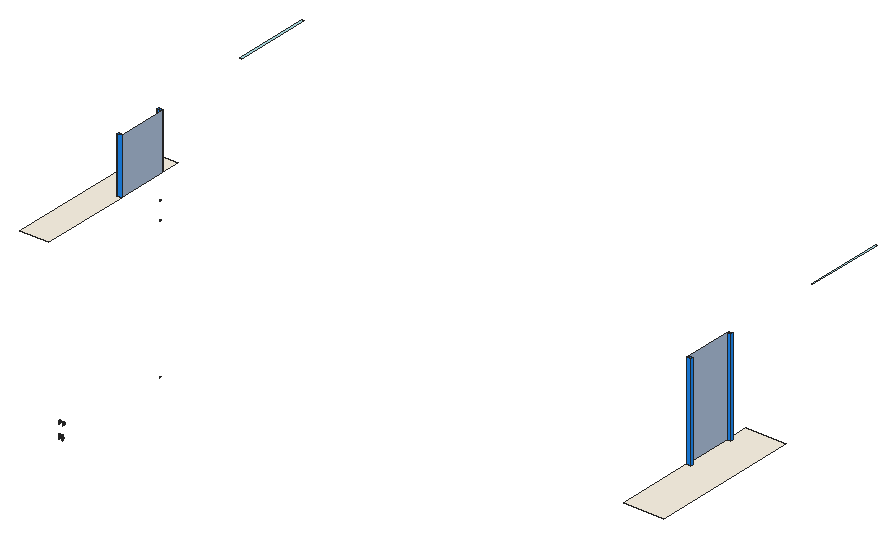
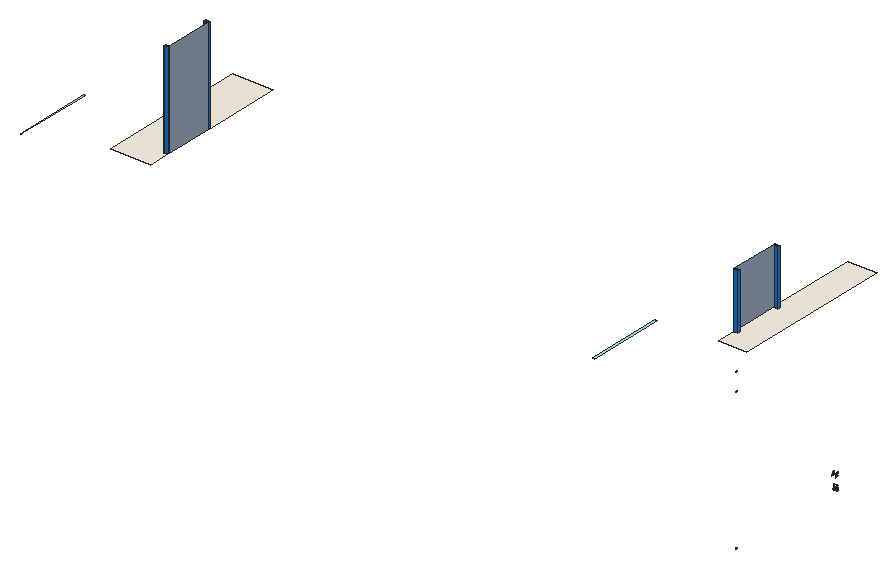
# SketchUp Ruby script. Lengths in inches.
U = 1.inch
M = Sketchup.active_model
def pt(a) = Geom::Point3d.new(a.map { |v| v * U })
def face(e, loops, mat)
  f = e.add_face(loops[0].map { |a| pt(a) })
  loops[1..].each { |l| e.add_face(l.map { |a| pt(a) }).erase! }
  f.material = f.back_material = mat if mat
  f
end
# faces: each face lists its corners as indices into pts; further lists are holes
def faces(e, pts, list, mat = nil) = list.each { |f| face(e, (f[0].is_a?(Array) ? f : [f]).map { |l| l.map { |i| pts[i] } }, mat) }
# xy, xz, yz: faces in a plane at the given z, y or x. An outline is a flat list of corners, or four numbers for a rectangle; further outlines are holes
def ring(l) = l.size == 4 ? [[l[0], l[1]], [l[2], l[1]], [l[2], l[3]], [l[0], l[3]]] : l.each_slice(2).to_a
def flat(e, list, mat, &to3) = list.each { |f| face(e, (f[0].is_a?(Array) ? f : [f]).map { |l| ring(l).map { |u, v| to3.(u, v) } }, mat) }
def xy(e, z, list, mat = nil) = flat(e, list, mat) { |x, y| [x, y, z] }
def xz(e, y, list, mat = nil) = flat(e, list, mat) { |x, z| [x, y, z] }
def yz(e, x, list, mat = nil) = flat(e, list, mat) { |y, z| [x, y, z] }
def lines(e, pts, list) = list.each { |a, b| e.add_line(pt(pts[a]), pt(pts[b])) }
# prism: a flat outline (further loops are holes) pulled along v
def prism(e, loops, v, mat = nil)
  f = face(e, loops, mat); d = Geom::Vector3d.new(v.map { |x| x * U })
  f.pushpull(f.normal.samedirection?(d) ? d.length : -d.length)
end
def box(e, o, s, mat = nil) = prism(e, [[o, [o[0] + s[0], o[1], o[2]], [o[0] + s[0], o[1] + s[1], o[2]], [o[0], o[1] + s[1], o[2]]]], [0, 0, s[2]], mat)
def at(x, y, z, deg = 0) = Geom::Transformation.translation(pt([x, y, z])) * Geom::Transformation.rotation(ORIGIN, Z_AXIS, deg.degrees)
def axes(o, x, y, z) = Geom::Transformation.new([*x, 0, *y, 0, *z, 0, *pt(o).to_a, 1])
def part(name) = M.definitions.add(name)
# library, detail: a bought-in or finely detailed component or shape, given as its bounding box
def library(name, o, s) = part(name).tap { |d| box(d.entities, o, s) }
def detail(e, o, s) = box(e.add_group.entities, o, s)
def put(e, d, t, mat = nil) = e.add_instance(d, t).tap { |i| i.material = mat if mat }
def group(e, t, mat = nil) = e.add_group.tap { |g| g.transformation = t; g.material = mat if mat }.entities
root = M.entities
M.materials.add("Material \#1").color = [140, 140, 140]
M.materials.add("[0030_OldLace]").color = [253, 245, 230]
M.materials.add("[0094_PowderBlue]").color = [176, 224, 230]
M.materials.add("[0098_DodgerBlue]").color = [30, 144, 255]
M.materials.add("[0099_LightSteelBlue]").color = [176, 196, 222]
xy(root,58.6641,[[266.1811,291.2578,266.1811,291.2765,266.1568,291.2691],[266.1811,291.2578,266.203,291.2867,266.1811,291.2765],[266.1811,291.2578,266.2055,291.2691,266.203,291.2867],[266.1568,291.2691,266.1593,291.2867,266.1355,291.3016],[266.1568,291.2691,266.1811,291.2765,266.1593,291.2867],
  [266.2055,291.2691,266.2223,291.316,266.203,291.2867],[266.2055,291.2691,266.2268,291.3016,266.2223,291.316],[266.1593,291.2867,266.14,291.316,266.1355,291.3016],[266.1355,291.3016,266.14,291.316,266.1196,291.3515],[266.2268,291.3016,266.2366,291.3609,266.2223,291.316],
  [266.2268,291.3016,266.2427,291.3515,266.2366,291.3609],[266.14,291.316,266.1257,291.3609,266.1196,291.3515],[266.1196,291.3515,266.1257,291.3609,266.1111,291.4127],[266.2427,291.3515,266.2441,291.4159,266.2366,291.3609],[266.2427,291.3515,266.2512,291.4127,266.2441,291.4159],
  [266.1257,291.3609,266.1181,291.4159,266.1111,291.4127],[266.1111,291.4127,266.1181,291.4159,266.1111,291.4778],[266.2512,291.4127,266.2442,291.4745,266.2441,291.4159],[266.2512,291.4127,266.2512,291.4778,266.2442,291.4745],[266.1181,291.4159,266.1181,291.4745,266.1111,291.4778],
  [266.1181,291.4745,266.1196,291.539,266.1111,291.4778],[266.1181,291.4745,266.1257,291.5296,266.1196,291.539],[266.2442,291.4745,266.2512,291.4778,266.2366,291.5296],[266.2512,291.4778,266.2427,291.539,266.2366,291.5296],[266.1257,291.5296,266.1355,291.5888,266.1196,291.539],
  [266.1257,291.5296,266.14,291.5745,266.1355,291.5888],[266.2366,291.5296,266.2427,291.539,266.2223,291.5745],[266.2427,291.539,266.2268,291.5888,266.2223,291.5745],[266.14,291.5745,266.1568,291.6214,266.1355,291.5888],[266.14,291.5745,266.1593,291.6038,266.1568,291.6214],
  [266.2223,291.5745,266.2268,291.5888,266.203,291.6038],[266.2268,291.5888,266.2055,291.6214,266.203,291.6038],[266.1593,291.6038,266.1811,291.6327,266.1568,291.6214],[266.1593,291.6038,266.1811,291.6139,266.1811,291.6327],[266.203,291.6038,266.2055,291.6214,266.1811,291.6139],
  [266.1811,291.6139,266.2055,291.6214,266.1811,291.6327]],"Material \#1")
xy(root,58.6839,[[266.1811,291.2578,266.1568,291.2691,266.1593,291.2867],[266.1811,291.2578,266.1593,291.2867,266.1811,291.2765],[266.1811,291.2578,266.1811,291.2765,266.2055,291.2691],[266.1568,291.2691,266.1355,291.3016,266.14,291.316],[266.1568,291.2691,266.14,291.316,266.1593,291.2867],
  [266.2055,291.2691,266.1811,291.2765,266.203,291.2867],[266.2055,291.2691,266.203,291.2867,266.2268,291.3016],[266.203,291.2867,266.2223,291.316,266.2268,291.3016],[266.1355,291.3016,266.1196,291.3515,266.1257,291.3609],[266.1355,291.3016,266.1257,291.3609,266.14,291.316],
  [266.2268,291.3016,266.2223,291.316,266.2427,291.3515],[266.2223,291.316,266.2366,291.3609,266.2427,291.3515],[266.1196,291.3515,266.1111,291.4127,266.1181,291.4159],[266.1196,291.3515,266.1181,291.4159,266.1257,291.3609],[266.2427,291.3515,266.2366,291.3609,266.2512,291.4127],
  [266.2366,291.3609,266.2441,291.4159,266.2512,291.4127],[266.1111,291.4127,266.1111,291.4778,266.1181,291.4745],[266.1111,291.4127,266.1181,291.4745,266.1181,291.4159],[266.2512,291.4127,266.2441,291.4159,266.2512,291.4778],[266.2441,291.4159,266.2442,291.4745,266.2512,291.4778],
  [266.1181,291.4745,266.1111,291.4778,266.1257,291.5296],[266.2442,291.4745,266.2366,291.5296,266.2427,291.539],[266.2442,291.4745,266.2427,291.539,266.2512,291.4778],[266.1111,291.4778,266.1196,291.539,266.1257,291.5296],[266.1257,291.5296,266.1196,291.539,266.14,291.5745],
  [266.2366,291.5296,266.2223,291.5745,266.2268,291.5888],[266.2366,291.5296,266.2268,291.5888,266.2427,291.539],[266.1196,291.539,266.1355,291.5888,266.14,291.5745],[266.14,291.5745,266.1355,291.5888,266.1593,291.6038],[266.2223,291.5745,266.203,291.6038,266.2055,291.6214],
  [266.2223,291.5745,266.2055,291.6214,266.2268,291.5888],[266.1355,291.5888,266.1568,291.6214,266.1593,291.6038],[266.1593,291.6038,266.1568,291.6214,266.1811,291.6139],[266.203,291.6038,266.1811,291.6139,266.1811,291.6327],[266.203,291.6038,266.1811,291.6327,266.2055,291.6214],
  [266.1811,291.6139,266.1568,291.6214,266.1811,291.6327]],"Material \#1")
xy(root,93.8273,[[266.1811,291.2578,266.1593,291.2867,266.1568,291.2691],[266.1811,291.2578,266.1811,291.2765,266.1593,291.2867],[266.1811,291.2578,266.2055,291.2691,266.1811,291.2765],[266.1568,291.2691,266.14,291.316,266.1355,291.3016],[266.1568,291.2691,266.1593,291.2867,266.14,291.316],
  [266.2055,291.2691,266.203,291.2867,266.1811,291.2765],[266.2055,291.2691,266.2268,291.3016,266.203,291.2867],[266.203,291.2867,266.2268,291.3016,266.2223,291.316],[266.1355,291.3016,266.1257,291.3609,266.1196,291.3515],[266.1355,291.3016,266.14,291.316,266.1257,291.3609],
  [266.2268,291.3016,266.2427,291.3515,266.2223,291.316],[266.2223,291.316,266.2427,291.3515,266.2365,291.3609],[266.1196,291.3515,266.1181,291.4159,266.1111,291.4127],[266.1196,291.3515,266.1257,291.3609,266.1181,291.4159],[266.2427,291.3515,266.2511,291.4127,266.2365,291.3609],
  [266.2365,291.3609,266.2511,291.4127,266.2441,291.4159],[266.1111,291.4127,266.1181,291.4159,266.1181,291.4745],[266.1111,291.4127,266.1181,291.4745,266.1111,291.4778],[266.2511,291.4127,266.2511,291.4778,266.2441,291.4159],[266.2441,291.4159,266.2511,291.4778,266.2441,291.4745],
  [266.1181,291.4745,266.1257,291.5296,266.1111,291.4778],[266.2441,291.4745,266.2427,291.539,266.2365,291.5296],[266.2441,291.4745,266.2511,291.4778,266.2427,291.539],[266.1111,291.4778,266.1257,291.5296,266.1196,291.539],[266.1257,291.5296,266.14,291.5745,266.1196,291.539],
  [266.2365,291.5296,266.2268,291.5888,266.2223,291.5745],[266.2365,291.5296,266.2427,291.539,266.2268,291.5888],[266.1196,291.539,266.14,291.5745,266.1355,291.5888],[266.14,291.5745,266.1593,291.6038,266.1355,291.5888],[266.2223,291.5745,266.2055,291.6214,266.203,291.6038],
  [266.2223,291.5745,266.2268,291.5888,266.2055,291.6214],[266.1355,291.5888,266.1593,291.6038,266.1568,291.6214],[266.1593,291.6038,266.1811,291.6139,266.1568,291.6214],[266.203,291.6038,266.1811,291.6327,266.1811,291.6139],[266.203,291.6038,266.2055,291.6214,266.1811,291.6327],
  [266.1811,291.6139,266.1811,291.6327,266.1568,291.6214]],"Material \#1")
xy(root,93.8471,[[266.1811,291.2578,266.1568,291.2691,266.1811,291.2765],[266.1811,291.2578,266.1811,291.2765,266.203,291.2867],[266.1811,291.2578,266.203,291.2867,266.2055,291.2691],[266.1568,291.2691,266.1355,291.3016,266.1593,291.2867],[266.1568,291.2691,266.1593,291.2867,266.1811,291.2765],
  [266.2055,291.2691,266.203,291.2867,266.2223,291.316],[266.2055,291.2691,266.2223,291.316,266.2268,291.3016],[266.1593,291.2867,266.1355,291.3016,266.14,291.316],[266.1355,291.3016,266.1196,291.3515,266.14,291.316],[266.2268,291.3016,266.2223,291.316,266.2365,291.3609],
  [266.2268,291.3016,266.2365,291.3609,266.2427,291.3515],[266.14,291.316,266.1196,291.3515,266.1257,291.3609],[266.1196,291.3515,266.1111,291.4127,266.1257,291.3609],[266.2427,291.3515,266.2365,291.3609,266.2441,291.4159],[266.2427,291.3515,266.2441,291.4159,266.2511,291.4127],
  [266.1257,291.3609,266.1111,291.4127,266.1181,291.4159],[266.1111,291.4127,266.1111,291.4778,266.1181,291.4159],[266.2511,291.4127,266.2441,291.4159,266.2441,291.4745],[266.2511,291.4127,266.2441,291.4745,266.2511,291.4778],[266.1181,291.4159,266.1111,291.4778,266.1181,291.4745],
  [266.1181,291.4745,266.1111,291.4778,266.1196,291.539],[266.1181,291.4745,266.1196,291.539,266.1257,291.5296],[266.2441,291.4745,266.2365,291.5296,266.2511,291.4778],[266.2511,291.4778,266.2365,291.5296,266.2427,291.539],[266.1257,291.5296,266.1196,291.539,266.1355,291.5888],
  [266.1257,291.5296,266.1355,291.5888,266.14,291.5745],[266.2365,291.5296,266.2223,291.5745,266.2427,291.539],[266.2427,291.539,266.2223,291.5745,266.2268,291.5888],[266.14,291.5745,266.1355,291.5888,266.1568,291.6214],[266.14,291.5745,266.1568,291.6214,266.1593,291.6038],
  [266.2223,291.5745,266.203,291.6038,266.2268,291.5888],[266.2268,291.5888,266.203,291.6038,266.2055,291.6214],[266.1593,291.6038,266.1568,291.6214,266.1811,291.6327],[266.1593,291.6038,266.1811,291.6327,266.1811,291.6139],[266.203,291.6038,266.1811,291.6139,266.2055,291.6214],
  [266.1811,291.6139,266.1811,291.6327,266.2055,291.6214]],"Material \#1")
xy(root,96,[[410,257.0899,410,276.9647,411,276.9647,411,277.4688,410,277.4688,410,289.4649,411,289.4649,411,289.9649,410,289.9649,410,295.4649,420,295.4649,420,257.0899]],"[0030_OldLace]")
xy(root,98.2902,[[266.1811,291.2578,266.1811,291.2765,266.1568,291.2691],[266.1811,291.2578,266.203,291.2867,266.1811,291.2765],[266.1811,291.2578,266.2055,291.2691,266.203,291.2867],[266.1568,291.2691,266.1593,291.2867,266.1355,291.3016],[266.1568,291.2691,266.1811,291.2765,266.1593,291.2867],
  [266.2055,291.2691,266.2223,291.316,266.203,291.2867],[266.2055,291.2691,266.2268,291.3016,266.2223,291.316],[266.1593,291.2867,266.14,291.316,266.1355,291.3016],[266.1355,291.3016,266.14,291.316,266.1196,291.3515],[266.2268,291.3016,266.2365,291.3609,266.2223,291.316],
  [266.2268,291.3016,266.2427,291.3515,266.2365,291.3609],[266.14,291.316,266.1257,291.3609,266.1196,291.3515],[266.1196,291.3515,266.1257,291.3609,266.1111,291.4127],[266.2427,291.3515,266.2441,291.4159,266.2365,291.3609],[266.2427,291.3515,266.2511,291.4127,266.2441,291.4159],
  [266.1257,291.3609,266.1181,291.4159,266.1111,291.4127],[266.1111,291.4127,266.1181,291.4159,266.1111,291.4778],[266.2511,291.4127,266.2441,291.4745,266.2441,291.4159],[266.2511,291.4127,266.2511,291.4778,266.2441,291.4745],[266.1181,291.4159,266.1181,291.4745,266.1111,291.4778],
  [266.1181,291.4745,266.1196,291.539,266.1111,291.4778],[266.1181,291.4745,266.1257,291.5296,266.1196,291.539],[266.2441,291.4745,266.2511,291.4778,266.2365,291.5296],[266.2511,291.4778,266.2427,291.539,266.2365,291.5296],[266.1257,291.5296,266.1355,291.5888,266.1196,291.539],
  [266.1257,291.5296,266.14,291.5745,266.1355,291.5888],[266.2365,291.5296,266.2427,291.539,266.2223,291.5745],[266.2427,291.539,266.2268,291.5888,266.2223,291.5745],[266.14,291.5745,266.1568,291.6214,266.1355,291.5888],[266.14,291.5745,266.1593,291.6038,266.1568,291.6214],
  [266.2223,291.5745,266.2268,291.5888,266.203,291.6038],[266.2268,291.5888,266.2055,291.6214,266.203,291.6038],[266.1593,291.6038,266.1811,291.6327,266.1568,291.6214],[266.1593,291.6038,266.1811,291.6139,266.1811,291.6327],[266.203,291.6038,266.2055,291.6214,266.1811,291.6139],
  [266.1811,291.6139,266.2055,291.6214,266.1811,291.6327]],"Material \#1")
xy(root,98.3101,[[266.1811,291.2578,266.1568,291.2691,266.1593,291.2867],[266.1811,291.2578,266.1593,291.2867,266.1811,291.2765],[266.1811,291.2578,266.1811,291.2765,266.2055,291.2691],[266.1568,291.2691,266.1355,291.3016,266.14,291.316],[266.1568,291.2691,266.14,291.316,266.1593,291.2867],
  [266.2055,291.2691,266.1811,291.2765,266.203,291.2867],[266.2055,291.2691,266.203,291.2867,266.2268,291.3016],[266.203,291.2867,266.2223,291.316,266.2268,291.3016],[266.1355,291.3016,266.1196,291.3515,266.1257,291.3609],[266.1355,291.3016,266.1257,291.3609,266.14,291.316],
  [266.2268,291.3016,266.2223,291.316,266.2427,291.3515],[266.2223,291.316,266.2365,291.3609,266.2427,291.3515],[266.1196,291.3515,266.1111,291.4127,266.1181,291.4159],[266.1196,291.3515,266.1181,291.4159,266.1257,291.3609],[266.2427,291.3515,266.2365,291.3609,266.2511,291.4127],
  [266.2365,291.3609,266.2441,291.4159,266.2511,291.4127],[266.1111,291.4127,266.1111,291.4778,266.1181,291.4745],[266.1111,291.4127,266.1181,291.4745,266.1181,291.4159],[266.2511,291.4127,266.2441,291.4159,266.2511,291.4778],[266.2441,291.4159,266.2441,291.4745,266.2511,291.4778],
  [266.1181,291.4745,266.1111,291.4778,266.1257,291.5296],[266.2441,291.4745,266.2365,291.5296,266.2427,291.539],[266.2441,291.4745,266.2427,291.539,266.2511,291.4778],[266.1111,291.4778,266.1196,291.539,266.1257,291.5296],[266.1257,291.5296,266.1196,291.539,266.14,291.5745],
  [266.2365,291.5296,266.2223,291.5745,266.2268,291.5888],[266.2365,291.5296,266.2268,291.5888,266.2427,291.539],[266.1196,291.539,266.1355,291.5888,266.14,291.5745],[266.14,291.5745,266.1355,291.5888,266.1593,291.6038],[266.2223,291.5745,266.203,291.6038,266.2055,291.6214],
  [266.2223,291.5745,266.2055,291.6214,266.2268,291.5888],[266.1355,291.5888,266.1568,291.6214,266.1593,291.6038],[266.1593,291.6038,266.1568,291.6214,266.1811,291.6139],[266.203,291.6038,266.1811,291.6139,266.1811,291.6327],[266.203,291.6038,266.1811,291.6327,266.2055,291.6214],
  [266.1811,291.6139,266.1568,291.6214,266.1811,291.6327]],"Material \#1")
xy(root,106,[[261,254.1412,261,294.632,268.125,294.632,268.125,289.9649,267,289.9649,267,289.4649,268.125,289.4649,268.125,277.4649,267,277.4649,267,276.9649,268.125,276.9649,268.125,254.1412]],"[0030_OldLace]")
xy(root,120,[[410.75,315.2149,411,334.9649],[267,315.4649,267.4375,334.9649]],"[0094_PowderBlue]")
xz(root,260.5367,[[265.6224,58.5031,265.7546,58.5031,265.6224,58.5378],[265.7546,58.5031,265.7546,58.5378,265.6224,58.5378],[266.3518,58.5031,266.484,58.5031,266.484,58.5378],[266.3518,58.5031,266.484,58.5378,266.3518,58.5378]],"Material \#1")
xz(root,260.5421,[[265.7546,58.3347,265.7546,58.3991,265.6224,58.3991],[266.3518,58.3347,266.484,58.3991,266.3518,58.3991]],"Material \#1")
xz(root,260.545,[[265.6224,58.447,265.7546,58.447,265.6224,58.475],[265.7546,58.447,265.7546,58.475,265.6224,58.475],[266.3518,58.447,266.484,58.447,266.484,58.475],[266.3518,58.447,266.484,58.475,266.3518,58.475]],"Material \#1")
xz(root,276.9647,[[410,96,411,120]],"[0098_DodgerBlue]")
xz(root,276.9649,[[267,106,268.125,120]],"[0098_DodgerBlue]")
xz(root,277.4649,[[267,106,268.125,120]],"[0098_DodgerBlue]")
xz(root,277.4688,[[410,96,411,120]],"[0098_DodgerBlue]")
xz(root,289.4649,[[410,96,411,120],[267,106,268.125,120]],"[0098_DodgerBlue]")
xz(root,289.9649,[[410,96,411,120],[267,106,268.125,120]],"[0098_DodgerBlue]")
yz(root,265.6267,[[260.5148,58.1118,260.5148,58.1514,260.5663,58.1593],[260.5148,58.1118,260.5663,58.1593,260.6136,58.1816],[260.5148,58.1118,260.6136,58.1816,260.7137,58.238],[260.5148,58.1118,260.6268,58.1461,260.5732,58.1207],[260.5148,58.1118,260.7137,58.238,260.6268,58.1461],
  [260.6268,58.1461,260.7137,58.238,260.6742,58.1858],[260.6136,58.1816,260.6554,58.2168,260.7137,58.238],[260.6554,58.2168,260.6903,58.2628,260.7137,58.238],[260.7137,58.238,260.6903,58.2628,260.7168,58.318],[260.7137,58.238,260.7168,58.318,260.7674,58.493],
  [260.7137,58.238,260.763,58.3714,260.7438,58.3006],[260.7137,58.238,260.7674,58.493,260.763,58.3714],[260.7168,58.318,260.7338,58.3805,260.7674,58.493],[260.763,58.3714,260.7674,58.493,260.7697,58.4486],[260.7338,58.3805,260.7397,58.4486,260.7674,58.493],
  [260.7397,58.4486,260.7338,58.5167,260.7674,58.493],[260.7674,58.493,260.663,58.7279,260.6662,58.7218],[260.7674,58.493,260.7168,58.5792,260.663,58.7279],[260.7674,58.493,260.6662,58.7218,260.6701,58.716],[260.7674,58.493,260.6701,58.716,260.7181,58.6488],
  [260.7674,58.493,260.7338,58.5167,260.7168,58.5792],[260.7674,58.493,260.7181,58.6488,260.75,58.5757],[260.7674,58.493,260.75,58.5757,260.7607,58.5354],[260.75,58.5757,260.7181,58.6488,260.7357,58.6136],[260.7168,58.5792,260.6903,58.6344,260.663,58.7279],
  [260.6903,58.6344,260.6554,58.6805,260.6587,58.7414],[260.6903,58.6344,260.6587,58.7414,260.663,58.7279],[260.7181,58.6488,260.6701,58.716,260.6746,58.7104],[260.7181,58.6488,260.6746,58.7104,260.6976,58.6812],[260.6554,58.6805,260.6136,58.7156,260.6572,59.1173],
  [260.6554,58.6805,260.6572,58.7572,260.6587,58.7414],[260.6554,58.6805,260.6572,59.1173,260.6572,58.7572],[260.6136,58.7156,260.5663,58.738,260.6572,59.1173],[260.663,58.7279,260.6587,58.7414,260.6605,58.7344],[260.4632,58.738,260.6259,59.235,260.5148,58.7458],
  [260.5663,58.738,260.5148,58.7458,260.6572,59.1173],[260.6587,58.7414,260.6572,58.7572,260.6576,58.749],[260.5148,58.7458,260.6259,59.235,260.6572,59.1173],[260.6572,59.1173,260.6259,59.235,260.6535,59.1604],[260.6535,59.1604,260.6259,59.235,260.6427,59.2],
  [260.6259,59.235,260.5148,59.3055,260.5774,59.2864],[260.6259,59.235,260.5774,59.2864,260.6038,59.2641],[260.5774,59.2864,260.5148,59.3055,260.5474,59.3005]],"Material \#1")
yz(root,265.6409,[[261.1596,61.4144,261.1488,61.5737,261.1599,61.5764],[261.1596,61.4144,261.1599,61.5764,261.1709,61.415],[260.5537,61.4841,260.5148,61.4944,260.5517,61.4987],[260.5537,61.4841,260.5517,61.4987,260.5907,61.4975],[260.5907,61.4975,260.5517,61.4987,260.5868,61.5115],
  [260.5907,61.4975,260.5868,61.5115,260.6247,61.5189],[260.5868,61.5115,260.619,61.5317,260.6247,61.5189],[260.6247,61.5189,260.619,61.5317,260.6551,61.5472],[260.619,61.5317,260.6478,61.5587,260.6551,61.5472],[260.6551,61.5472,260.6478,61.5587,260.6813,61.5819],
  [260.6478,61.5587,260.6727,61.5915,260.6813,61.5819],[261.1488,61.5737,261.1189,61.7175,261.1294,61.7227],[261.1488,61.5737,261.1294,61.7227,261.1599,61.5764],[260.6813,61.5819,260.6727,61.5915,260.7028,61.622],[260.6727,61.5915,260.6931,61.6295,260.7028,61.622],
  [260.7028,61.622,260.6931,61.6295,260.719,61.667],[260.6931,61.6295,260.7084,61.6722,260.719,61.667],[260.719,61.667,260.7084,61.6722,260.7291,61.7158],[260.7084,61.6722,260.718,61.7185,260.7291,61.7158],[260.7291,61.7158,260.718,61.7185,260.7326,61.7673],
  [261.1189,61.7175,261.0712,61.85,261.0809,61.8576],[261.1189,61.7175,261.0809,61.8576,261.1294,61.7227],[260.718,61.7185,260.7213,61.7673,260.7326,61.7673],[260.7213,61.7673,260.718,61.8161,260.7291,61.8188],[260.7213,61.7673,260.7291,61.8188,260.7326,61.7673],
  [260.718,61.8161,260.7084,61.8624,260.719,61.8676],[260.718,61.8161,260.719,61.8676,260.7291,61.8188],[261.0712,61.85,261.0076,61.9689,261.0162,61.9785],[261.0712,61.85,261.0162,61.9785,261.0809,61.8576],[260.7084,61.8624,260.6931,61.905,260.7028,61.9126],
  [260.7084,61.8624,260.7028,61.9126,260.719,61.8676],[260.6931,61.905,260.6727,61.9431,260.6813,61.9527],[260.6931,61.905,260.6813,61.9527,260.7028,61.9126],[260.6727,61.9431,260.6478,61.9759,260.6551,61.9873],[260.6727,61.9431,260.6551,61.9873,260.6813,61.9527],
  [261.0076,61.9689,260.9298,62.0717,260.9371,62.0831],[261.0076,61.9689,260.9371,62.0831,261.0162,61.9785],[260.6478,61.9759,260.619,62.0028,260.6247,62.0157],[260.6478,61.9759,260.6247,62.0157,260.6551,61.9873],[260.619,62.0028,260.5868,62.0231,260.5907,62.0371],
  [260.619,62.0028,260.5907,62.0371,260.6247,62.0157],[260.5868,62.0231,260.5517,62.0358,260.5537,62.0505],[260.5868,62.0231,260.5537,62.0505,260.5907,62.0371],[260.5517,62.0358,260.5148,62.0551,260.5537,62.0505],[260.9298,62.0717,260.8398,62.1557,260.8455,62.1686],
  [260.9298,62.0717,260.8455,62.1686,260.9371,62.0831],[260.8398,62.1557,260.7395,62.2187,260.7435,62.2327],[260.8398,62.1557,260.7435,62.2327,260.8455,62.1686],[260.7395,62.2187,260.6307,62.2582,260.6327,62.2729],[260.7395,62.2187,260.6327,62.2729,260.7435,62.2327],
  [260.6307,62.2582,260.5148,62.272,260.5148,62.2869],[260.6307,62.2582,260.5148,62.2869,260.6327,62.2729]],"Material \#1")
yz(root,265.7688,[[260.5148,58.1118,260.5663,58.1593,260.5148,58.1514],[260.5148,58.1118,260.5732,58.1207,260.6268,58.1461],[260.5148,58.1118,260.6136,58.1816,260.5663,58.1593],[260.5148,58.1118,260.6268,58.1461,260.7137,58.238],[260.5148,58.1118,260.7137,58.238,260.6136,58.1816],
  [260.6268,58.1461,260.6742,58.1858,260.7137,58.238],[260.6136,58.1816,260.7137,58.238,260.6554,58.2168],[260.6554,58.2168,260.7137,58.238,260.6903,58.2628],[260.7137,58.238,260.7168,58.318,260.6903,58.2628],[260.7137,58.238,260.7338,58.3805,260.7168,58.318],
  [260.7137,58.238,260.7438,58.3006,260.763,58.3714],[260.7137,58.238,260.763,58.3714,260.7674,58.493],[260.7137,58.238,260.7674,58.493,260.7338,58.3805],[260.763,58.3714,260.7697,58.4486,260.7674,58.493],[260.7338,58.3805,260.7674,58.493,260.7397,58.4486],
  [260.7397,58.4486,260.7674,58.493,260.7338,58.5167],[260.7674,58.493,260.663,58.7279,260.6903,58.6344],[260.7674,58.493,260.6662,58.7218,260.663,58.7279],[260.7674,58.493,260.6701,58.716,260.6662,58.7218],[260.7674,58.493,260.7181,58.6488,260.6701,58.716],
  [260.7674,58.493,260.6903,58.6344,260.7168,58.5792],[260.7674,58.493,260.7168,58.5792,260.7338,58.5167],[260.7674,58.493,260.75,58.5757,260.7181,58.6488],[260.7674,58.493,260.7607,58.5354,260.75,58.5757],[260.75,58.5757,260.7357,58.6136,260.7181,58.6488],
  [260.6903,58.6344,260.663,58.7279,260.6554,58.6805],[260.7181,58.6488,260.6746,58.7104,260.6701,58.716],[260.7181,58.6488,260.6976,58.6812,260.6746,58.7104],[260.6554,58.6805,260.663,58.7279,260.6136,58.7156],[260.6136,58.7156,260.663,58.7279,260.5663,58.738],
  [260.663,58.7279,260.6587,58.7414,260.5663,58.738],[260.663,58.7279,260.6605,58.7344,260.6587,58.7414],[260.3668,58.7285,260.6572,59.1173,260.6535,59.1604],[260.4632,58.738,260.5148,58.7458,260.6572,59.1173],[260.5663,58.738,260.6572,59.1173,260.5148,58.7458],
  [260.5663,58.738,260.6572,58.7572,260.6572,59.1173],[260.5663,58.738,260.6587,58.7414,260.6572,58.7572],[260.6587,58.7414,260.6576,58.749,260.6572,58.7572],[260.6535,59.1604,260.5774,59.2864,260.4521,59.2864],[260.6535,59.1604,260.6259,59.235,260.5774,59.2864],
  [260.6535,59.1604,260.6427,59.2,260.6259,59.235],[260.6259,59.235,260.6038,59.2641,260.5774,59.2864],[260.5774,59.2864,260.5474,59.3005,260.5148,59.3055]],"Material \#1")
yz(root,266.3375,[[260.5148,58.1118,260.5148,58.1514,260.5663,58.1593],[260.5148,58.1118,260.5663,58.1593,260.6136,58.1816],[260.5148,58.1118,260.6136,58.1816,260.7137,58.238],[260.5148,58.1118,260.6268,58.1461,260.5732,58.1207],[260.5148,58.1118,260.7137,58.238,260.6268,58.1461],
  [260.6268,58.1461,260.7137,58.238,260.6742,58.1858],[260.6136,58.1816,260.6554,58.2168,260.7137,58.238],[260.6554,58.2168,260.6903,58.2628,260.7137,58.238],[260.7137,58.238,260.6903,58.2628,260.7168,58.318],[260.7137,58.238,260.7168,58.318,260.7338,58.3805],
  [260.7137,58.238,260.7338,58.3805,260.7674,58.493],[260.7137,58.238,260.763,58.3714,260.7438,58.3006],[260.7137,58.238,260.7674,58.493,260.763,58.3714],[260.763,58.3714,260.7674,58.493,260.7697,58.4486],[260.7338,58.3805,260.7397,58.4486,260.7674,58.493],
  [260.7397,58.4486,260.7338,58.5167,260.7674,58.493],[260.7674,58.493,260.663,58.7279,260.6662,58.7218],[260.7674,58.493,260.6903,58.6344,260.663,58.7279],[260.7674,58.493,260.6662,58.7218,260.6701,58.716],[260.7674,58.493,260.6701,58.716,260.7181,58.6488],
  [260.7674,58.493,260.7168,58.5792,260.6903,58.6344],[260.7674,58.493,260.7338,58.5167,260.7168,58.5792],[260.7674,58.493,260.7181,58.6488,260.75,58.5757],[260.7674,58.493,260.75,58.5757,260.7607,58.5354],[260.75,58.5757,260.7181,58.6488,260.7357,58.6136],
  [260.6903,58.6344,260.6554,58.6805,260.663,58.7279],[260.7181,58.6488,260.6701,58.716,260.6746,58.7104],[260.7181,58.6488,260.6746,58.7104,260.6976,58.6812],[260.6554,58.6805,260.6136,58.7156,260.663,58.7279],[260.6136,58.7156,260.5663,58.738,260.663,58.7279],
  [260.663,58.7279,260.5663,58.738,260.6587,58.7414],[260.663,58.7279,260.6587,58.7414,260.6605,58.7344],[260.3668,58.7285,260.6535,59.1604,260.6572,59.1173],[260.4632,58.738,260.6572,59.1173,260.5148,58.7458],[260.5663,58.738,260.5148,58.7458,260.6572,59.1173],
  [260.5663,58.738,260.6572,58.7572,260.6587,58.7414],[260.5663,58.738,260.6572,59.1173,260.6572,58.7572],[260.6587,58.7414,260.6572,58.7572,260.6576,58.749],[260.6535,59.1604,260.4521,59.2864,260.5774,59.2864],[260.6535,59.1604,260.5774,59.2864,260.6259,59.235],
  [260.6535,59.1604,260.6259,59.235,260.6427,59.2],[260.6259,59.235,260.5774,59.2864,260.6038,59.2641],[260.5774,59.2864,260.5148,59.3055,260.5474,59.3005]],"Material \#1")
yz(root,266.4655,[[261.1596,61.4144,261.1599,61.5764,261.1488,61.5737],[261.1596,61.4144,261.1709,61.415,261.1599,61.5764],[260.5537,61.4841,260.5517,61.4988,260.5148,61.4944],[260.5537,61.4841,260.5907,61.4975,260.5517,61.4988],[260.5907,61.4975,260.5868,61.5115,260.5517,61.4988],
  [260.5907,61.4975,260.6247,61.5189,260.5868,61.5115],[260.5868,61.5115,260.6247,61.5189,260.619,61.5317],[260.6247,61.5189,260.6551,61.5472,260.619,61.5317],[260.619,61.5317,260.6551,61.5472,260.6478,61.5587],[260.6551,61.5472,260.6813,61.5819,260.6478,61.5587],
  [260.6478,61.5587,260.6813,61.5819,260.6727,61.5915],[261.1488,61.5737,261.1294,61.7227,261.1189,61.7175],[261.1488,61.5737,261.1599,61.5764,261.1294,61.7227],[260.6813,61.5819,260.7028,61.622,260.6727,61.5915],[260.6727,61.5915,260.7028,61.622,260.6931,61.6295],
  [260.7028,61.622,260.719,61.667,260.6931,61.6295],[260.6931,61.6295,260.719,61.667,260.7084,61.6722],[260.719,61.667,260.7291,61.7158,260.7084,61.6722],[260.7084,61.6722,260.7291,61.7158,260.718,61.7185],[260.7291,61.7158,260.7326,61.7673,260.718,61.7185],
  [261.1189,61.7175,261.0809,61.8576,261.0712,61.85],[261.1189,61.7175,261.1294,61.7227,261.0809,61.8576],[260.718,61.7185,260.7326,61.7673,260.7213,61.7673],[260.7213,61.7673,260.7291,61.8188,260.718,61.8161],[260.7213,61.7673,260.7326,61.7673,260.7291,61.8188],
  [260.718,61.8161,260.719,61.8676,260.7084,61.8624],[260.718,61.8161,260.7291,61.8188,260.719,61.8676],[261.0712,61.85,261.0162,61.9785,261.0076,61.9689],[261.0712,61.85,261.0809,61.8576,261.0162,61.9785],[260.7084,61.8624,260.7028,61.9126,260.6931,61.905],
  [260.7084,61.8624,260.719,61.8676,260.7028,61.9126],[260.6931,61.905,260.6813,61.9527,260.6727,61.9431],[260.6931,61.905,260.7028,61.9126,260.6813,61.9527],[260.6727,61.9431,260.6551,61.9873,260.6478,61.9759],[260.6727,61.9431,260.6813,61.9527,260.6551,61.9873],
  [261.0076,61.9689,260.9371,62.0831,260.9298,62.0717],[261.0076,61.9689,261.0162,61.9785,260.9371,62.0831],[260.6478,61.9759,260.6247,62.0157,260.619,62.0029],[260.6478,61.9759,260.6551,61.9873,260.6247,62.0157],[260.619,62.0029,260.5907,62.0371,260.5868,62.0231],
  [260.619,62.0029,260.6247,62.0157,260.5907,62.0371],[260.5868,62.0231,260.5537,62.0505,260.5517,62.0358],[260.5868,62.0231,260.5907,62.0371,260.5537,62.0505],[260.5517,62.0358,260.5537,62.0505,260.5148,62.0551],[260.9298,62.0717,260.8455,62.1686,260.8398,62.1557],
  [260.9298,62.0717,260.9371,62.0831,260.8455,62.1686],[260.8398,62.1557,260.7435,62.2327,260.7395,62.2187],[260.8398,62.1557,260.8455,62.1686,260.7435,62.2327],[260.7395,62.2187,260.6327,62.2729,260.6307,62.2582],[260.7395,62.2187,260.7435,62.2327,260.6327,62.2729],
  [260.6307,62.2582,260.5148,62.2869,260.5148,62.272],[260.6307,62.2582,260.6327,62.2729,260.5148,62.2869]],"Material \#1")
yz(root,266.4797,[[260.5148,58.1118,260.5663,58.1593,260.5148,58.1514],[260.5148,58.1118,260.5732,58.1207,260.6268,58.1461],[260.5148,58.1118,260.6136,58.1816,260.5663,58.1593],[260.5148,58.1118,260.6268,58.1461,260.7137,58.238],[260.5148,58.1118,260.7137,58.238,260.6136,58.1816],
  [260.6268,58.1461,260.6742,58.1858,260.7137,58.238],[260.6136,58.1816,260.7137,58.238,260.6554,58.2168],[260.6554,58.2168,260.7137,58.238,260.6903,58.2628],[260.7137,58.238,260.7168,58.318,260.6903,58.2628],[260.7137,58.238,260.7438,58.3006,260.763,58.3714],
  [260.7137,58.238,260.763,58.3714,260.7674,58.493],[260.7137,58.238,260.7674,58.493,260.7168,58.318],[260.7168,58.318,260.7674,58.493,260.7338,58.3805],[260.763,58.3714,260.7697,58.4486,260.7674,58.493],[260.7338,58.3805,260.7674,58.493,260.7397,58.4486],
  [260.7397,58.4486,260.7674,58.493,260.7338,58.5167],[260.7674,58.493,260.663,58.7279,260.7168,58.5792],[260.7674,58.493,260.6662,58.7218,260.663,58.7279],[260.7674,58.493,260.6701,58.716,260.6662,58.7218],[260.7674,58.493,260.7181,58.6488,260.6701,58.716],
  [260.7674,58.493,260.7168,58.5792,260.7338,58.5167],[260.7674,58.493,260.75,58.5757,260.7181,58.6488],[260.7674,58.493,260.7607,58.5354,260.75,58.5757],[260.75,58.5757,260.7357,58.6136,260.7181,58.6488],[260.7168,58.5792,260.663,58.7279,260.6903,58.6344],
  [260.3393,58.6344,260.3741,58.6805,260.6259,59.235],[260.6903,58.6344,260.6587,58.7414,260.6554,58.6805],[260.6903,58.6344,260.663,58.7279,260.6587,58.7414],[260.7181,58.6488,260.6746,58.7104,260.6701,58.716],[260.7181,58.6488,260.6976,58.6812,260.6746,58.7104],
  [260.3741,58.6805,260.4159,58.7156,260.6259,59.235],[260.6554,58.6805,260.6572,59.1173,260.6136,58.7156],[260.6554,58.6805,260.6572,58.7572,260.6572,59.1173],[260.6554,58.6805,260.6587,58.7414,260.6572,58.7572],[260.6136,58.7156,260.6572,59.1173,260.5663,58.738],
  [260.663,58.7279,260.6605,58.7344,260.6587,58.7414],[260.3668,58.7285,260.6259,59.235,260.3693,58.7352],[260.3693,58.7352,260.6259,59.235,260.371,58.7422],[260.4632,58.738,260.5148,58.7458,260.6259,59.235],[260.5663,58.738,260.6572,59.1173,260.5148,58.7458],
  [260.6587,58.7414,260.6576,58.749,260.6572,58.7572],[260.371,58.7422,260.6259,59.235,260.372,58.7495],[260.5148,58.7458,260.6572,59.1173,260.6259,59.235],[260.6572,59.1173,260.6535,59.1604,260.6259,59.235],[260.6535,59.1604,260.6427,59.2,260.6259,59.235],
  [260.6259,59.235,260.5774,59.2864,260.5148,59.3055],[260.6259,59.235,260.6038,59.2641,260.5774,59.2864],[260.5774,59.2864,260.5474,59.3005,260.5148,59.3055]],"Material \#1")
yz(root,267,[[276.9649,106,277.4649,120],[289.4649,106,289.9649,120]],"[0098_DodgerBlue]")
yz(root,268.125,[[277.4649,106,289.4649,120]],"[0099_LightSteelBlue]")
yz(root,410,[[277.4688,96,289.4649,120]],"[0099_LightSteelBlue]")
yz(root,411,[[276.9647,96,277.4688,120],[289.4649,96,289.9649,120]],"[0098_DodgerBlue]")
p = [[265.7546,260.5421,58.2505],[265.7546,260.5421,58.3149],[265.6224,260.5392,58.3226],[265.6224,260.5392,58.3226],[265.6224,260.5421,58.2505],[265.7546,260.5421,58.2505],
  [265.6224,260.5421,58.3991],[265.6224,260.5392,58.3226],[265.7546,260.5421,58.3347],[266.484,260.5392,58.3226],[266.3518,260.5421,58.3149],[266.3518,260.5421,58.2505],
  [266.3518,260.5421,58.2505],[266.484,260.5421,58.2505],[266.484,260.5392,58.3226],[266.3518,260.5421,58.3347],[266.484,260.5392,58.3226],[266.484,260.5421,58.3991],
  [265.7546,260.5421,58.3991],[265.7546,260.5367,58.4189],[265.6224,260.5367,58.4189],[265.6224,260.545,58.447],[265.6224,260.5367,58.4189],[265.7546,260.5367,58.4189],
  [265.6224,260.5367,58.4189],[265.6224,260.5421,58.3991],[265.7546,260.5421,58.3991],[265.7546,260.5367,58.4189],[265.7546,260.545,58.447],[265.6224,260.545,58.447],
  [266.484,260.5367,58.4189],[266.3518,260.5367,58.4189],[266.3518,260.5421,58.3991],[266.3518,260.5367,58.4189],[266.484,260.5367,58.4189],[266.484,260.545,58.447],
  [266.3518,260.5421,58.3991],[266.484,260.5421,58.3991],[266.484,260.5367,58.4189],[266.484,260.545,58.447],[266.3518,260.545,58.447],[266.3518,260.5367,58.4189],
  [265.7546,260.5367,58.5378],[265.7546,260.5259,58.5749],[265.6224,260.5287,58.5799],[265.6224,260.5287,58.5799],[265.6224,260.5367,58.5378],[265.7546,260.5367,58.5378],
  [265.6224,260.5367,58.5031],[265.6224,260.545,58.475],[265.7546,260.545,58.475],[265.7546,260.5367,58.5031],[266.484,260.5287,58.5799],[266.3518,260.5259,58.5749],
  [266.3518,260.5367,58.5378],[266.3518,260.5367,58.5378],[266.484,260.5367,58.5378],[266.484,260.5287,58.5799],[266.484,260.5367,58.5031],[266.3518,260.5367,58.5031],
  [266.3518,260.545,58.475],[266.3518,260.545,58.475],[266.484,260.545,58.475],[266.484,260.5367,58.5031],[265.6224,260.5287,58.6121],[265.6224,260.5287,58.5799],
  [265.7546,260.5316,58.5848],[265.7546,260.5316,58.6071],[265.6224,260.5367,58.6467],[265.6224,260.5287,58.6121],[265.7546,260.5259,58.617],[265.7546,260.5259,58.617],
  [265.7546,260.5367,58.6467],[265.6224,260.5367,58.6467],[266.484,260.5287,58.6121],[266.3518,260.5316,58.6071],[266.3518,260.5316,58.5848],[266.484,260.5287,58.5799],
  [266.3518,260.5259,58.617],[266.484,260.5287,58.6121],[266.484,260.5367,58.6467],[266.484,260.5367,58.6467],[266.3518,260.5367,58.6467],[266.3518,260.5259,58.617]]
faces(root,p,[[0,1,2],[3,4,5],[6,7,8],[9,10,11],[12,13,14],[15,16,17],[18,19,20],[21,22,23],
  [24,25,26],[27,28,29],[30,31,32],[33,34,35],[36,37,38],[39,40,41],[42,43,44],[45,46,47],
  [48,49,50],[50,51,48],[52,53,54],[55,56,57],[58,59,60],[61,62,63],[64,65,66],[66,67,64],
  [68,69,70],[71,72,73],[74,75,76],[76,77,74],[78,79,80],[81,82,83]],"Material \#1")
